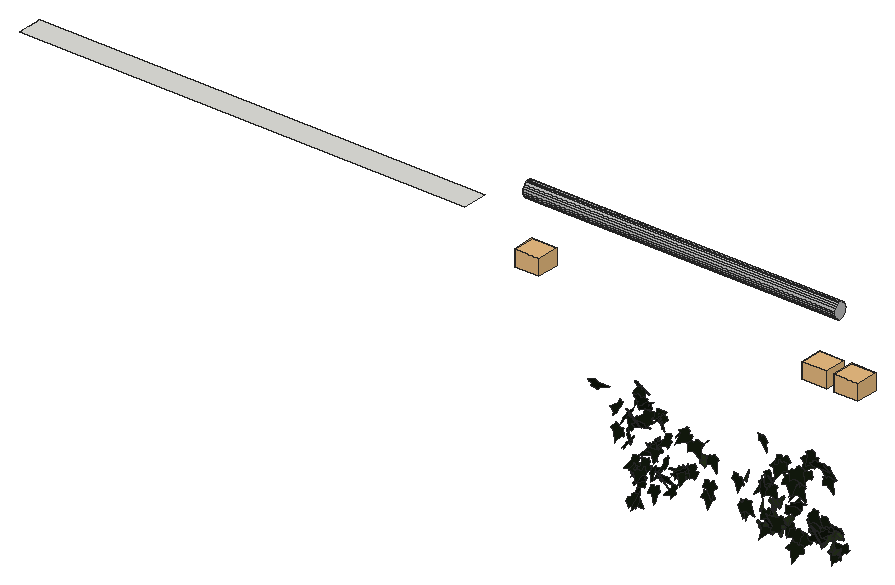
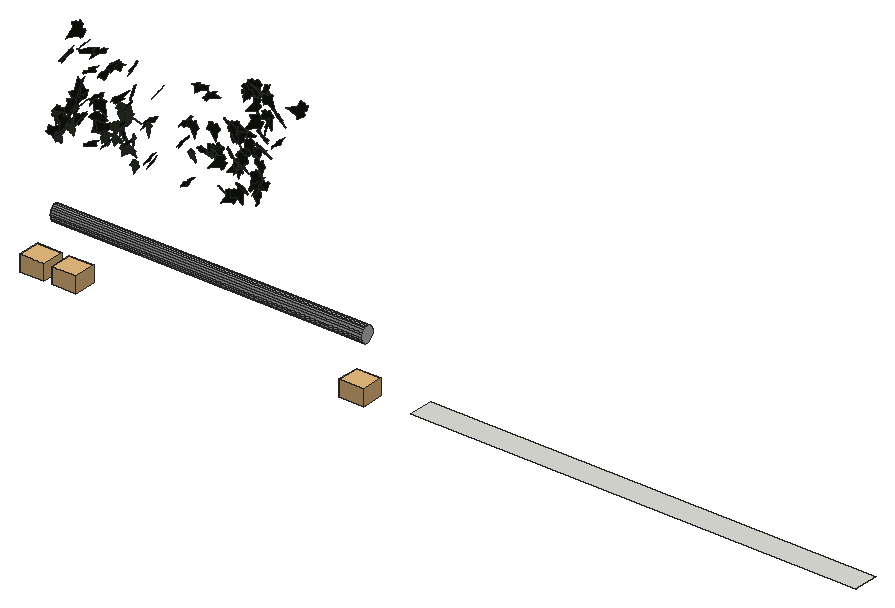
# SketchUp Ruby script. Lengths in inches.
U = 1.inch
M = Sketchup.active_model
def pt(a) = Geom::Point3d.new(a.map { |v| v * U })
def face(e, loops, mat)
  f = e.add_face(loops[0].map { |a| pt(a) })
  loops[1..].each { |l| e.add_face(l.map { |a| pt(a) }).erase! }
  f.material = f.back_material = mat if mat
  f
end
# faces: each face lists its corners as indices into pts; further lists are holes
def faces(e, pts, list, mat = nil) = list.each { |f| face(e, (f[0].is_a?(Array) ? f : [f]).map { |l| l.map { |i| pts[i] } }, mat) }
# xy, xz, yz: faces in a plane at the given z, y or x. An outline is a flat list of corners, or four numbers for a rectangle; further outlines are holes
def ring(l) = l.size == 4 ? [[l[0], l[1]], [l[2], l[1]], [l[2], l[3]], [l[0], l[3]]] : l.each_slice(2).to_a
def flat(e, list, mat, &to3) = list.each { |f| face(e, (f[0].is_a?(Array) ? f : [f]).map { |l| ring(l).map { |u, v| to3.(u, v) } }, mat) }
def xy(e, z, list, mat = nil) = flat(e, list, mat) { |x, y| [x, y, z] }
def xz(e, y, list, mat = nil) = flat(e, list, mat) { |x, z| [x, y, z] }
def yz(e, x, list, mat = nil) = flat(e, list, mat) { |y, z| [x, y, z] }
def lines(e, pts, list) = list.each { |a, b| e.add_line(pt(pts[a]), pt(pts[b])) }
# prism: a flat outline (further loops are holes) pulled along v
def prism(e, loops, v, mat = nil)
  f = face(e, loops, mat); d = Geom::Vector3d.new(v.map { |x| x * U })
  f.pushpull(f.normal.samedirection?(d) ? d.length : -d.length)
end
def box(e, o, s, mat = nil) = prism(e, [[o, [o[0] + s[0], o[1], o[2]], [o[0] + s[0], o[1] + s[1], o[2]], [o[0], o[1] + s[1], o[2]]]], [0, 0, s[2]], mat)
def at(x, y, z, deg = 0) = Geom::Transformation.translation(pt([x, y, z])) * Geom::Transformation.rotation(ORIGIN, Z_AXIS, deg.degrees)
def axes(o, x, y, z) = Geom::Transformation.new([*x, 0, *y, 0, *z, 0, *pt(o).to_a, 1])
def part(name) = M.definitions.add(name)
# library, detail: a bought-in or finely detailed component or shape, given as its bounding box
def library(name, o, s) = part(name).tap { |d| box(d.entities, o, s) }
def detail(e, o, s) = box(e.add_group.entities, o, s)
def put(e, d, t, mat = nil) = e.add_instance(d, t).tap { |i| i.material = mat if mat }
def group(e, t, mat = nil) = e.add_group.tap { |g| g.transformation = t; g.material = mat if mat }.entities
root = M.entities
M.materials.add("Glass Rail Metal").color = [192, 192, 192]
M.materials.add("[Translucent Glass Tinted]").color = [8, 201, 241]
M.materials["[Translucent Glass Tinted]"].alpha = 0.48
M.materials.add("efeu1").color = [18, 25, 13]
M.materials.add("efeu2").color = [43, 57, 29]
c1 = library("glass bracket3",[-2.83,-0.98,-1],[3.67,3.29,2])
c2 = part("ivyleaf_9")
p = [[1.54,2.16,1.25],[1.36,2.04,1.19],[-0.21,0.99,0.68],[-0.71,1.11,0.82],[-0.85,0.86,0.67],[-0.8,0.17,0.21],
  [-0.9,-0.01,0.1],[-0.67,-0.16,-0.02],[-0.08,-0.08,-0.05],[-0.03,-0.6,-0.4],[0.65,-0.88,-0.66],[0.83,-0.6,-0.49],
  [1.29,-0.42,-0.43],[1.8125,-0.07,-0.26],[1.21,0.44,0.15]]
faces(c2.entities,p,[[0,1,2,3,4,5,6,7,8,9,10,11,12,13,14]],"efeu1")
c3 = library("glass bracket3\#1",[-0.84,-0.98,-1],[3.67,3.29,2])
c4 = part("ivyleaf_10")
p = [[0,0.5,-0.03],[-0.0625,2.02,-0.43],[-0.19,2.01,-0.46],[-0.54,1.05,-0.29],[-0.52,0.625,-0.18],[-0.83,0.76,-0.28],
  [-1.16,0.64,-0.33],[-1.15,0.33,-0.24],[-0.77,-0.39,0.02],[-0.3,-0.51,0.16],[0.04,-0.48,0.23],[-0.02,2.01,-0.4375],
  [-0.06,2.01,-0.43],[0.04,-0.49,0.23],[0.67,-0.49,0.14],[1.38,0.36,-0.2],[1.375,0.51,-0.24],[0.81,0.65,-0.19],
  [0.62,0.59,-0.15],[0.6,1.09,-0.28],[0.5,1.23,-0.31]]
faces(c4.entities,p,[[0,1,2,3,4,5,6,7,8,9,10],[11,12,0,13,14,15,16,17,18,19,20]],"efeu2")
prism(root,[[[415.35,180.51,322.8],[415.35,180.12,323.16],[415.35,179.8125,323.625],[415.35,179.625,324.17],[415.35,179.56,324.75],[415.35,179.625,325.34],[415.35,179.8125,325.88],[415.35,180.12,326.35],[415.35,180.51,326.71],[415.35,180.97,326.9375],[415.35,181.46,327.01],[415.35,181.95,326.9375],[415.35,182.41,326.71],[415.35,182.8,326.35],[415.35,183.1,325.88],[415.35,183.29,325.34],[415.35,183.36,324.75],[415.35,183.29,324.17],[415.35,183.1,323.625],[415.35,182.8,323.16],[415.35,182.41,322.8],[415.35,181.95,322.57],[415.35,181.46,322.49],[415.35,180.97,322.57]]],[89.11,0,0],"Glass Rail Metal")
xy(root,313.73,[[270.09,181.4375,270.19,188.5625],[270.19,181.4375,397.3,188.5625]])
put(root,c1,axes([420.75,178.46,309.14],[1.9,0,0],[0,1.9,0],[0,0,2.261]),"[Translucent Glass Tinted]")
put(root,c2,axes([485.94,116.3,328.26],[0.8101,-0.2449,1.09923],[1.12749,-0.18692,-0.81555],[0.31902,1.28251,0.09104]))
put(root,c2,axes([493.41,115.95,324.74],[-0.65893,0.94328,0.65335],[-0.47886,0.45794,-1.16294],[-1.12644,-0.74646,0.11218]))
put(root,c2,axes([492.45,117.625,318.39],[-0.28136,-1.15514,0.46252],[-0.09169,-0.43673,-1.23145],[1.33367,-0.27372,0.01291]))
put(root,c2,axes([495.57,118.78,319.65],[-0.17105,0.55401,1.19106],[-0.80611,0.89413,-0.55718],[-1.11267,-0.73295,0.22057]))
put(root,c2,axes([494.75,121.1,329.17],[1.23153,-0.34226,0.23288],[0.22972,-0.07027,-1.23817],[0.37729,1.15996,-0.00629]))
put(root,c2,axes([496.13,122.76,319.99],[-0.45959,1.04403,-0.33265],[0.17313,-0.27984,-1.17174],[-1.16651,-0.45287,-0.04284]))
put(root,c2,axes([497.27,117.82,302.66],[-0.00432,-0.15519,1.32579],[0.41697,1.21568,0.15517],[-1.32278,0.38372,0.04458]))
put(root,c2,axes([497.75,119.7,306.05],[-0.20946,-1.14874,-0.3107],[0.04515,-0.30914,1.20799],[-1.28111,0.17692,0.09337]))
put(root,c2,axes([497.77,114.01,320.44],[0.78084,-0.24418,-1.0962],[-1.0422,0.42774,-0.79146],[0.52842,1.20447,0.05884]))
put(root,c2,axes([498.27,124.44,307.27],[-0.05681,1.00946,-0.51276],[-0.33082,-0.48776,-1.00462],[-1.16733,0.0891,0.30967]))
put(root,c2,axes([498.58,123.58,314.36],[-1.02751,0.63409,-0.14789],[0.02451,-0.21954,-1.17605],[-0.7014,-0.93658,0.17555]))
put(root,c2,axes([498.58,113.24,326.47],[-0.59445,1.0226,-0.56708],[0.21124,-0.51302,-1.20593],[-1.23365,-0.5806,0.06677]))
put(root,c2,axes([498.73,115.64,310.64],[-0.2863,1.17234,0.39649],[-0.12539,0.36448,-1.24959],[-1.32547,-0.2877,0.03257]))
put(root,c2,axes([498.44,121.83,314.83],[0.28495,1.07624,0.44218],[0.0195,0.43221,-1.14944],[-1.2496,0.25216,0.0829]))
put(root,c2,axes([498.22,116.83,307.59],[0.51596,1.00158,0.57895],[0.26454,0.49992,-1.15406],[-1.20895,0.53685,-0.00544]))
put(root,c2,axes([498.01,116.8,321.99],[1.1703,0.49825,0.45385],[0.38527,0.26598,-1.23707],[-0.6027,1.1375,0.09047]))
put(root,c2,axes([498.89,117.28,330.47],[-1.12566,-0.2867,-0.62392],[0.69335,-0.14357,-1.08862],[0.18692,-1.194,0.28071]))
put(root,c2,axes([499.95,114.6,313.75],[-1.26982,0.472,0.31035],[-0.2989,0.1116,-1.31764],[-0.52381,-1.20789,-0.00047]))
put(root,c2,axes([498.86,114.17,304.44],[0.17341,-0.52438,-1.23481],[-0.13475,1.18459,-0.56165],[1.3953,0.17958,0.09922]))
put(root,c2,axes([500.14,111.25,320.61],[-0.35999,1.24725,-0.17607],[0.0476,-0.16346,-1.34266],[-1.35855,-0.33622,-0.00039]))
put(root,c2,axes([500.28,122.55,322.01],[-0.12628,1.21383,-0.03725],[0.00924,-0.03515,-1.26821],[-1.31147,-0.11712,-0.00535]))
put(root,c2,axes([500.83,122.77,322.5],[-0.20605,-0.13622,-1.23794],[-0.77863,-0.94962,0.2332],[-1.03345,0.74263,0.07112]))
put(root,c2,axes([499.15,112.71,327.07],[1.09918,-0.76749,0.25485],[0.21787,-0.13947,-1.32565],[0.8424,1.03751,0.01032]))
put(root,c2,axes([500.55,115.24,330.125],[0.71667,0.52303,-1.00338],[-0.90602,-0.48513,-0.8736],[-0.76414,1.06574,0.09476]))
put(root,c2,axes([499.55,123.91,305.48],[1.18677,0.19902,0.31235],[0.32194,0.03922,-1.16132],[-0.21856,1.13849,-0.01459]))
put(root,c2,axes([500.59,122.86,319.25],[0.48986,-0.75362,0.85767],[-0.3052,0.78372,0.90648],[-1.16729,-0.52117,0.12291]))
put(root,c2,axes([499.41,119.78,314.94],[0.79145,-0.92996,0.50067],[0.3237,-0.37674,-1.23136],[1.08365,0.79174,0.00215]))
put(root,c2,axes([500.75,112.77,303.46],[-0.93903,0.85894,-0.29007],[-0.25797,0.15465,1.26973],[0.9406,0.89992,0.05865]))
put(root,c2,axes([500.57,114.68,312.42],[-0.68469,-1.07197,-0.13881],[0.0822,0.11004,-1.29519],[1.16377,-0.63845,0.00982]))
put(root,c2,axes([501.43,116.53,312.63],[-0.59556,-0.45756,1.02266],[-0.72892,-0.71874,-0.74145],[0.9169,-0.86859,0.07482]))
put(root,c3,axes([499.09,178.46,309.14],[1.9,0,0],[0,1.9,0],[0,0,2.261]),"[Translucent Glass Tinted]")
put(root,c2,axes([501.12,119.53,305.22],[-0.87342,-0.33977,-0.86946],[0.90569,0.13173,-0.89934],[0.36002,-1.15568,0.15311]))
put(root,c2,axes([501.45,115.11,328.6],[0.74871,1.0217,0.22928],[0.10976,0.19741,-1.28379],[-1.12348,0.70017,0.02738]))
put(root,c2,axes([502.63,118.48,309.35],[-0.12174,1.01264,0.66087],[-0.20284,0.61535,-1.05447],[-1.27512,-0.19457,0.10465]))
put(root,c2,axes([501.98,117.43,316.66],[0.30474,0.01748,1.22803],[0.85087,0.90159,-0.20967],[-0.95009,0.81305,0.20611]))
put(root,c2,axes([503.01,117.09,317.13],[-0.17027,-0.19232,-1.25547],[-0.1927,-1.20053,0.22315],[-1.30606,0.2022,0.13075]))
put(root,c2,axes([503.49,114.75,325.98],[-0.78878,-0.16042,1.08566],[-1.06641,-0.34671,-0.77387],[0.40481,-1.22595,0.0768]))
put(root,c2,axes([502.43,116.64,310.1],[-0.29372,0.763,1.00463],[0.22041,-0.94765,0.83821],[1.31106,0.33025,0.08416]))
put(root,c2,axes([503.01,117.34,317.4],[-0.39357,-1.16034,-0.20277],[0.06105,0.1866,-1.26486],[1.26926,-0.36877,-0.00203]))
put(root,c2,axes([502.63,118.9,309.57],[1.05577,-0.6977,0.14082],[0.11566,-0.08302,-1.24903],[0.75881,0.9834,-0.00554]))
put(root,c2,axes([504.6,122.1875,304.65],[-0.98898,0.64819,0.31507],[-0.29719,0.13515,-1.16577],[-0.7133,-0.95502,0.04887]))
put(root,c2,axes([504.52,119.4375,313.19],[-1.1026,0.54204,-0.36383],[0.33351,-0.1644,-1.20213],[-0.61174,-1.06661,0.00039]))
put(root,c2,axes([506.18,118.44,319.85],[-1.21661,0.43265,0.15191],[-0.14501,0.05779,-1.25497],[-0.47137,-1.13445,-0.006]))
put(root,c2,axes([504.99,120.97,310.92],[1.21351,0.13269,0.38591],[0.33046,0.41283,-1.11711],[-0.26822,1.10896,0.36968]))
put(root,c2,axes([506.42,122.53,320.27],[-0.16307,1.21085,0.02267],[-0.00236,0.0217,-1.26904],[-1.30793,-0.15101,-0.00054]))
put(root,c2,axes([508.72,118.96,312.51],[-0.06243,1.23409,-0.48109],[-0.19619,-0.46607,-1.26952],[-1.40979,0.01021,0.19798]))
put(root,c2,axes([509.27,119.875,311.43],[-1.00499,0.52956,0.75703],[-0.70113,0.33046,-1.11312],[-0.67346,-1.13428,0.02914]))
put(root,c2,axes([508.9375,119.84,312.63],[-0.50476,1.17635,0.04594],[-0.06746,0.02268,-1.31541],[-1.26956,-0.46891,0.05164]))
put(root,c2,axes([508.88,120.05,312.11],[-0.43001,-1.19105,0.1552],[0.07989,-0.18127,-1.2994],[1.29393,-0.38463,0.13181]))
put(root,c4,axes([510.52,125.63,313.27],[0.70864,-0.41175,-0.9334],[-0.80464,0.47307,-0.81957],[0.62715,1.0722,0.00316]))
put(root,c1,axes([511.95,178.46,309.14],[1.9,0,0],[0,1.9,0],[0,0,2.261]),"[Translucent Glass Tinted]")
put(root,c2,axes([510.95,121.42,312.34],[-1.23379,-0.0339,0.16638],[-0.16595,-0.01743,-1.23419],[0.03592,-1.24484,0.01275]))
put(root,c2,axes([512.08,117.64,323.75],[-0.82206,-0.78213,0.61308],[-0.46129,-0.40443,-1.13447],[0.88023,-0.94238,-0.02196]))
put(root,c2,axes([512.42,122.49,318.8],[-0.28114,1.23747,0.10978],[-0.02681,0.10649,-1.269],[-1.24204,-0.2824,0.00255]))
put(root,c2,axes([512.05,125.18,305.14],[-0.14885,-1.21491,0.03913],[-0.00939,-0.03827,-1.22399],[1.2155,-0.14907,-0.00467]))
put(root,c2,axes([513.3,124.74,315.04],[0.36887,-1.16725,-0.24276],[-0.02678,0.24593,-1.22322],[1.19193,0.36676,0.04764]))
put(root,c2,axes([516.05,115.02,323.96],[-0.31305,-0.87829,-0.93817],[0.69221,0.69832,-0.88473],[1.08278,-0.70037,0.29436]))
put(root,c2,axes([519.35,116.42,314.3125],[0.05795,-1.29748,-0.05119],[-0.00115,0.05119,-1.29877],[1.29849,0.05795,0.00114]))
put(root,c2,axes([522.39,124.97,306.125],[0.06296,-1.12647,0.5068],[0.00042,-0.50744,-1.12795],[1.23523,0.05759,-0.02545]))
put(root,c4,axes([523.78,124.23,314.88],[0.34007,-1.18371,-0.29161],[-0.00165,0.30229,-1.22901],[1.2191,0.33061,0.07968]))
put(root,c2,axes([523.54,124.29,306.54],[0.05571,-1.20049,0.29909],[0.01634,-0.29865,-1.20178],[1.23707,0.05801,0.0024]))
put(root,c4,axes([527.8125,123.8,303.72],[-1.17809,0.31352,0.14915],[-0.14718,0.02687,-1.21904],[-0.31444,-1.18719,0.0118]))
put(root,c2,axes([527.46,116.43,318.47],[0.10152,-1.20535,0.54246],[0.09857,-0.53564,-1.20865],[1.31811,0.13289,0.04861]))
put(root,c4,axes([528.82,123.18,309.57],[0.54598,-1.09409,-0.25622],[0.09842,0.33033,-1.20082],[1.11937,0.5046,0.23055]))
put(root,c2,axes([528.31,117.35,311.88],[0.45223,-0.89994,-0.83525],[0.00274,0.89084,-0.95835],[1.22781,0.32948,0.30978]))
put(root,c2,axes([529.75,123.27,314.9],[-1.25588,0.06796,-0.12555],[0.10454,-0.31928,-1.21851],[-0.09723,-1.22109,0.31161]))
put(root,c4,axes([530.1,124.13,315.5],[-0.41976,-1.18904,0.12701],[-0.01665,-0.12878,-1.26067],[1.19569,-0.41922,0.02703]))
put(root,c4,axes([530.1,123.33,316.63],[-1.17977,0.44528,0.13812],[-0.12349,0.06393,-1.2609],[-0.44956,-1.1861,-0.01611]))
put(root,c2,axes([529.34,122.5625,326.93],[0.56836,-1.14064,0.29714],[0.10361,-0.28026,-1.27401],[1.17414,0.57687,-0.03141]))
put(root,c2,axes([530.15,124.2,313.65],[0.32951,-1.03081,-0.64812],[0.1422,0.69941,-1.0401],[1.2093,0.19863,0.29891]))
put(root,c2,axes([530.27,122.92,308.04],[0.28987,-1.13046,-0.4308],[0.06762,0.45744,-1.15488],[1.20788,0.24569,0.16804]))
put(root,c2,axes([530.64,123.81,316.74],[-0.27921,-0.83368,0.91943],[-0.09744,-0.92478,-0.86812],[1.23729,-0.26096,0.13912]))
put(root,c2,axes([531.56,121.84,305.35],[-1.18193,-0.31854,-0.22534],[0.23608,-0.01147,-1.22203],[0.31066,-1.20317,0.07131]))
put(root,c4,axes([531.65,121.95,305.65],[-1.09726,-0.35053,-0.47335],[0.5076,-0.05507,-1.13588],[0.29879,-1.19374,0.1914]))
put(root,c2,axes([532.64,122.41,309.25],[-0.98289,0.60512,-0.4951],[0.43503,-0.23755,-1.15398],[-0.64965,-1.0746,-0.0237]))
put(root,c4,axes([533.39,123.99,311.67],[-0.16549,-1.23971,-0.1588],[0.0319,0.15594,-1.25065],[1.24943,-0.16818,0.0109]))
put(root,c2,axes([533.67,117.57,316.33],[-0.07496,-0.80622,1.06803],[0.11832,1.06152,0.80961],[-1.33292,0.13957,0.01181]))
put(root,c4,axes([533.96,121.02,310.22],[-1.08842,0.57265,0.29014],[-0.27446,0.10117,-1.22931],[-0.58033,-1.12187,0.03724]))
put(root,c4,axes([534.83,119.59,313.9],[-1.26043,0.13065,-0.07539],[0.07544,-0.00345,-1.26717],[-0.13063,-1.26268,-0.00433]))
put(root,c4,axes([534.92,121.62,306.79],[1.17134,0.08212,0.48523],[0.48161,0.06634,-1.17383],[-0.10121,1.26613,0.03003]))
put(root,c2,axes([535.67,124.48,306.23],[-0.1485,-1.1774,0.40813],[0.0093,-0.41205,-1.18534],[1.2461,-0.13724,0.05748]))
put(root,c4,axes([536.14,124.28,307.89],[-0.17814,-1.20198,0.33615],[-0.00349,-0.33908,-1.21429],[1.2481,-0.17251,0.04458]))
put(root,c2,axes([535.24,117.4,309.02],[0.33277,-0.5275,1.09837],[0.9352,-0.6193,-0.58075],[0.78107,0.96624,0.22741]))
put(root,c2,axes([536.54,124.21,309.47],[-0.64812,-0.16836,1.07496],[1.03096,0.30498,0.66936],[-0.34785,1.21761,-0.01902]))
put(root,c2,axes([536.51,121.07,324.67],[-0.02641,-1.34964,-0.23457],[-0.00199,0.23465,-1.34989],[1.36988,-0.02568,-0.00648]))
put(root,c2,axes([536.9,119.625,324.05],[-0.81244,-1.0034,-0.16955],[0.16835,0.08144,-1.28866],[1.00361,-0.82594,0.07891]))
put(root,c2,axes([538.35,123.5,315.69],[-0.32989,1.09644,-0.59269],[-0.01137,-0.61572,-1.13272],[-1.24633,-0.2846,0.16721]))
put(root,c2,axes([537.93,123.85,312.33],[0.87382,0.90991,-0.20544],[-0.22573,-0.06686,-1.2563],[-0.90509,0.89515,0.11499]))
put(root,c2,axes([538.89,123.49,316.97],[0.2809,-1.07826,-0.65282],[0.0226,0.67304,-1.10192],[1.26028,0.22826,0.16527]))
put(root,c2,axes([540.44,115.14,311.45],[-0.58731,-1.32292,-0.21243],[-0.08448,-0.19492,1.44743],[-1.3372,0.59335,0.00186]))
put(root,c2,axes([539.73,119.8,321.1],[-0.18779,-1.33126,-0.24343],[0.00986,0.24441,-1.34423],[1.3533,-0.18652,-0.02398]))
put(root,c2,axes([540.78,124.23,304.49],[-0.70398,-0.9991,0.2392],[0.00189,-0.29123,-1.21086],[1.02733,-0.6841,0.16614]))
put(root,c2,axes([540.78,120.28,307.78],[0.05292,-1.31287,-0.26727],[-0.02543,0.26644,-1.31386],[1.33956,0.05692,-0.01438]))
put(root,c2,axes([541.87,122.82,322.28],[-0.59344,-1.13866,0.25644],[0.01923,-0.29719,-1.27506],[1.16702,-0.57412,0.15142]))
put(root,c2,axes([542.51,118.61,305.28],[-0.79506,-1.08884,-0.15786],[0.09315,0.12745,-1.34822],[1.09628,-0.8005,0.00007]))
put(root,c2,axes([542.64,117.98,324.98],[0.13938,-1.08195,-0.8611],[0.3353,0.86608,-1.03393],[1.34152,-0.10406,0.34789]))
put(root,c2,axes([543.76,122.08,326.31],[-0.9374,-0.88542,0.28103],[-0.09576,-0.30503,-1.28042],[0.924,-0.92987,0.15242]))
put(root,c2,axes([544.3,122.38,327.27],[-0.5425,-0.88244,0.8236],[-0.03177,-0.8922,-0.97688],[1.20665,-0.42023,0.34456]))
put(root,c2,axes([544,122.64,308.82],[0.35944,-1.21451,-0.01669],[-0.00784,0.01509,-1.26658],[1.2146,0.35952,-0.00324]))
put(root,c2,axes([544.22,122.89,309.85],[0.19823,-1.10014,-0.58465],[0.03397,0.59656,-1.11103],[1.24538,0.15884,0.12336]))
put(root,c2,axes([545.05,120.88,313.56],[0.60596,-0.89399,-0.82884],[-0.31034,0.78197,-1.07032],[1.17893,0.66534,0.14427]))
put(root,c2,axes([544.92,120.9,311.875],[0.63675,-1.01359,-0.45084],[0.00739,0.52369,-1.16695],[1.10931,0.57832,0.26656]))
put(root,c2,axes([545.48,123.95,310.86],[0.95495,-0.67714,-0.50126],[-0.10781,0.65323,-1.08783],[0.83556,0.85818,0.43252]))
put(root,c4,axes([546.37,123.4,306.5625],[0.28284,-1.20646,0.1928],[0.06622,-0.18247,-1.23896],[1.21997,0.28962,0.02255]))
put(root,c2,axes([546.05,123.87,308.57],[0.09063,-1.2401,0.20466],[0.02544,-0.20334,-1.24337],[1.25662,0.09356,0.01041]))
put(root,c4,axes([547.09,123.88,307.25],[-0.70363,-0.91714,0.50176],[-0.06463,-0.56551,-1.12429],[1.04343,-0.65349,0.26872]))
put(root,c2,axes([547.24,124.4,308.96],[1.04021,0.55849,-0.37223],[-0.33163,-0.16923,-1.18063],[-0.58352,1.09177,0.00741]))
put(root,c2,axes([547.35,122.52,325.17],[0.98209,-0.69823,-0.53524],[-0.20441,0.59912,-1.15663],[0.8557,0.94448,0.338]))
put(root,c2,axes([548.22,119.96,309.56],[0.64162,0.78271,0.95793],[0.55736,0.78047,-1.01102],[-1.10436,0.84864,0.0463]))
put(root,c2,axes([547.93,118.07,328.75],[1.36208,0.27047,0.30087],[0.29285,0.06992,-1.38863],[-0.27914,1.39316,0.01128]))
put(root,c4,axes([549.21,124.63,308.69],[-0.00664,-1.25247,-0.04474],[-0.04637,0.04496,-1.25162],[1.25241,-0.00497,-0.04658]))
put(root,c4,axes([549.07,122.92,306.04],[0.37129,-1.07508,-0.53467],[0.09493,0.58418,-1.10871],[1.19693,0.28716,0.25379]))
put(root,c2,axes([548.6,121.99,323.41],[0.40331,-1.21333,-0.28459],[-0.02092,0.29249,-1.27665],[1.24608,0.39762,0.07068]))
put(root,c2,axes([549.16,123.88,309.98],[1.03954,0.34611,-0.58921],[-0.57438,-0.13857,-1.09476],[-0.37021,1.18685,0.04401]))
put(root,c4,axes([549.52,124.4375,303.76],[0.02174,-1.15734,0.43482],[0.01129,-0.43468,-1.15754],[1.23628,0.02432,0.00293]))
put(root,c2,axes([549.37,123.94,303.64],[-0.29332,-1.08127,0.51387],[0.04889,-0.53945,-1.10718],[1.19617,-0.24309,0.17126]))
put(root,c2,axes([550.43,125.01,303.93],[0.38617,0.00991,1.17737],[-1.16751,0.16357,0.38156],[-0.15237,-1.22824,0.06031]))
put(root,c2,axes([549.4375,116.45,310.2],[1.31007,0.3691,0.38071],[-0.3668,-0.10197,1.36107],[0.38293,-1.36045,0.00127]))
put(root,c4,axes([549.87,124.35,304.14],[0.95645,-0.74795,0.22627],[0.15243,-0.17218,-1.21349],[0.76642,0.96765,-0.04103]))
put(root,c4,axes([549.23,124.11,308.58],[-0.45223,-0.2196,-1.13518],[1.11232,-0.41535,-0.36277],[-0.3156,-1.14918,0.34804]))
put(root,c2,axes([550.51,116.26,310.74],[0.57185,-1.10328,0.69756],[-0.28042,0.63994,1.24204],[-1.27482,-0.63566,0.03969]))
